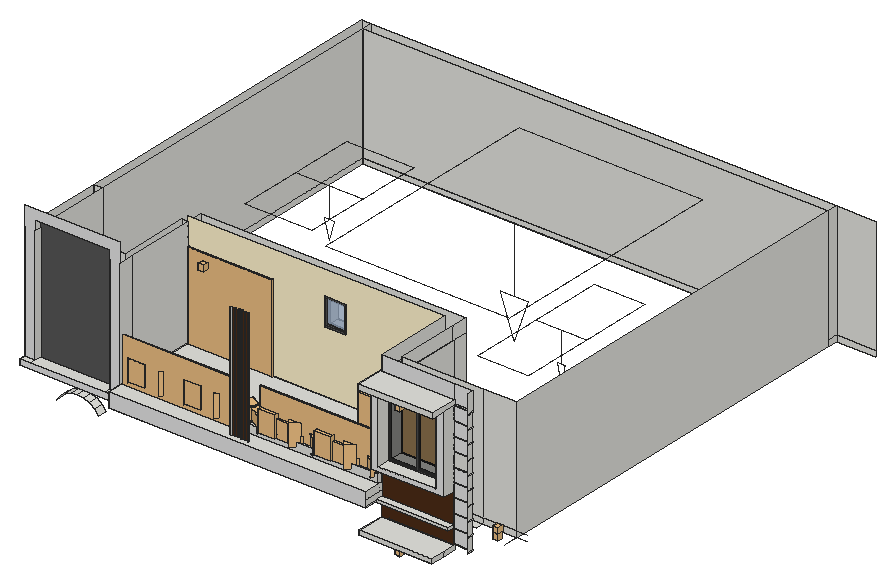
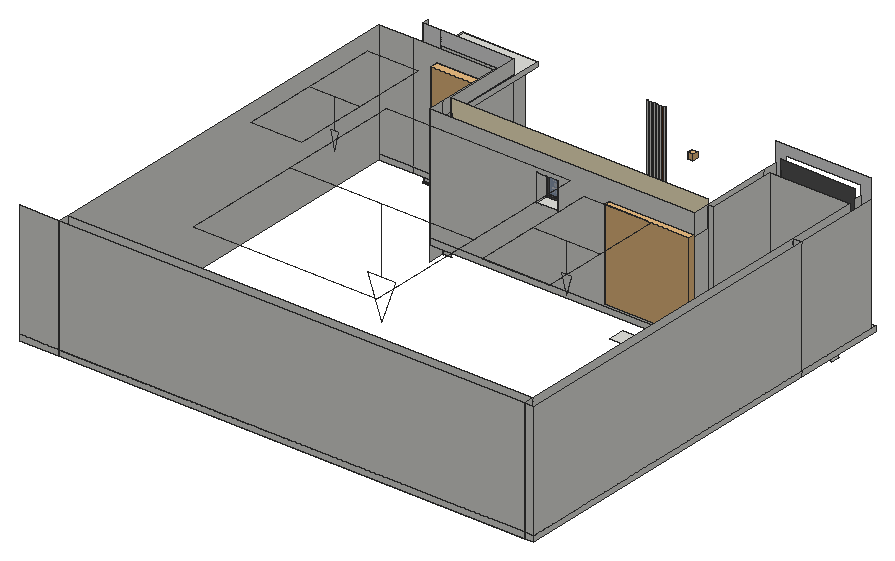
# SketchUp Ruby script. Lengths in inches.
U = 1.inch
M = Sketchup.active_model
def pt(a) = Geom::Point3d.new(a.map { |v| v * U })
def face(e, loops, mat)
  f = e.add_face(loops[0].map { |a| pt(a) })
  loops[1..].each { |l| e.add_face(l.map { |a| pt(a) }).erase! }
  f.material = f.back_material = mat if mat
  f
end
# faces: each face lists its corners as indices into pts; further lists are holes
def faces(e, pts, list, mat = nil) = list.each { |f| face(e, (f[0].is_a?(Array) ? f : [f]).map { |l| l.map { |i| pts[i] } }, mat) }
# xy, xz, yz: faces in a plane at the given z, y or x. An outline is a flat list of corners, or four numbers for a rectangle; further outlines are holes
def ring(l) = l.size == 4 ? [[l[0], l[1]], [l[2], l[1]], [l[2], l[3]], [l[0], l[3]]] : l.each_slice(2).to_a
def flat(e, list, mat, &to3) = list.each { |f| face(e, (f[0].is_a?(Array) ? f : [f]).map { |l| ring(l).map { |u, v| to3.(u, v) } }, mat) }
def xy(e, z, list, mat = nil) = flat(e, list, mat) { |x, y| [x, y, z] }
def xz(e, y, list, mat = nil) = flat(e, list, mat) { |x, z| [x, y, z] }
def yz(e, x, list, mat = nil) = flat(e, list, mat) { |y, z| [x, y, z] }
def lines(e, pts, list) = list.each { |a, b| e.add_line(pt(pts[a]), pt(pts[b])) }
# prism: a flat outline (further loops are holes) pulled along v
def prism(e, loops, v, mat = nil)
  f = face(e, loops, mat); d = Geom::Vector3d.new(v.map { |x| x * U })
  f.pushpull(f.normal.samedirection?(d) ? d.length : -d.length)
end
def box(e, o, s, mat = nil) = prism(e, [[o, [o[0] + s[0], o[1], o[2]], [o[0] + s[0], o[1] + s[1], o[2]], [o[0], o[1] + s[1], o[2]]]], [0, 0, s[2]], mat)
def at(x, y, z, deg = 0) = Geom::Transformation.translation(pt([x, y, z])) * Geom::Transformation.rotation(ORIGIN, Z_AXIS, deg.degrees)
def axes(o, x, y, z) = Geom::Transformation.new([*x, 0, *y, 0, *z, 0, *pt(o).to_a, 1])
def part(name) = M.definitions.add(name)
# library, detail: a bought-in or finely detailed component or shape, given as its bounding box
def library(name, o, s) = part(name).tap { |d| box(d.entities, o, s) }
def detail(e, o, s) = box(e.add_group.entities, o, s)
def put(e, d, t, mat = nil) = e.add_instance(d, t).tap { |i| i.material = mat if mat }
def group(e, t, mat = nil) = e.add_group.tap { |g| g.transformation = t; g.material = mat if mat }.entities
root = M.entities
M.materials.add("Glass_Tinted_Gray").color = [0, 0, 0]
M.materials["Glass_Tinted_Gray"].alpha = 0.125
M.materials.add("Material__1").color = [95, 70, 46]
M.materials.add("[0135_DarkGray]").color = [81, 81, 81]
M.materials.add("[Color D01]").color = [255, 242, 204]
M.materials.add("[Color M01]").color = [226, 226, 226]
M.materials.add("[Color M06]").color = [86, 86, 86]
M.materials.add("[Color_006]").color = [86, 86, 86]
M.materials.add("[Mirror 02]").color = [229, 229, 229]
M.materials.add("[Terrazzo Light Blue]").color = [196, 214, 227]
M.materials.add("[Translucent_Glass_Gray]1").color = [167, 187, 214]
M.materials["[Translucent_Glass_Gray]1"].alpha = 0.8
M.materials.add("[Wood Veneer 01]").color = [76, 44, 23]
c1 = library("SPOT",[0,0,1.68],[5.4375,5.4375,6.28])
c2 = library("Sliding Door",[0,0,0],[94.49,5.83,91.73])
c3 = library("Curtains",[0,0,0],[121.73,8.19,117.22])
c4 = part("glass-railing")
detail(c4.entities,[0,0,0],[1.26,75.59,33.1875])
c5 = library("Areca palm plant",[0,0,0],[49.1,36.6,54.46])
c6 = library("Group20\#1",[-20.81,-17.08,3.79],[39.86,39.43,37.51])
c7 = library("Group\#74",[-84.69,-90.07,-0.36],[176.51,175.13,171.4])
c8 = library("Group\#130",[-7.34,-1.2,0],[38.67,35.81,49.04])
c9 = library("Group38\#2",[14.01,28.44,-23.43],[18.58,18.32,38.89])
c10 = part("Group\#11")
put(c10.entities,c5,axes([-6.2,56.6,6.08],[0.45017,-0.56191,0],[0.66137,0.52986,0],[0,0,0.72]))
put(c10.entities,c5,axes([-6.2,158.41,6.08],[0.45017,-0.56191,0],[0.66137,0.52986,0],[0,0,0.72]))
put(c10.entities,c6,axes([18.97,181.79,4.77],[0,0.85,0],[-0.85,0,0],[0,0,0.85]))
put(c10.entities,c7,axes([14.93,71.3,6.05],[-0.04961,-0.08593,0],[0.08593,-0.04961,0],[0,0,0.10522]))
put(c10.entities,c7,axes([14.93,91.37,6.05],[-0.04961,-0.08593,0],[0.08593,-0.04961,0],[0,0,0.10522]))
put(c10.entities,c6,axes([18.97,79.98,4.77],[0,0.85,0],[-0.85,0,0],[0,0,0.85]))
put(c10.entities,c8,axes([24.9375,191.72,8],[0,0.79,0],[-0.79,0,0],[0,0,0.79]))
put(c10.entities,c7,axes([17.19,223.04,6.07],[-0.08133,-0.14087,0],[0.14087,-0.08133,0],[0,0,0.1725]))
put(c10.entities,c8,axes([24.9375,89.91,8],[0,0.79,0],[-0.79,0,0],[0,0,0.79]))
put(c10.entities,c7,axes([14.93,44.05,6.05],[-0.04961,-0.08593,0],[0.08593,-0.04961,0],[0,0,0.10522]))
put(c10.entities,c7,axes([14.93,145.87,6.05],[-0.04961,-0.08593,0],[0.08593,-0.04961,0],[0,0,0.10522]))
put(c10.entities,c9,axes([-4.1,100.66,28.17],[0.8848,0,0],[0,0.94674,0],[0,0,0.85826]))
put(c10.entities,c7,axes([14.93,173.12,6.05],[-0.04961,-0.08593,0],[0.08593,-0.04961,0],[0,0,0.10522]))
put(c10.entities,c9,axes([-4.1,-1.15,28.17],[0.8848,0,0],[0,0.94674,0],[0,0,0.85826]))
put(c10.entities,c7,axes([17.19,121.23,6.07],[-0.08133,-0.14087,0],[0.14087,-0.08133,0],[0,0,0.1725]))
put(c10.entities,c7,axes([14.93,193.18,6.05],[-0.04961,-0.08593,0],[0.08593,-0.04961,0],[0,0,0.10522]))
put(c10.entities,c7,axes([17.19,15.79,6.07],[-0.08133,-0.14087,0],[0.14087,-0.08133,0],[0,0,0.1725]))
g1 = group(c10.entities,at(0,0,0))
xy(g1,0,[[0,0,6,234.8],[30,0,36,234.8]])
xy(g1,3,[[6,0,30,234.8]])
xy(g1,7,[[6,5,30,229.8]],"Material__1")
xy(g1,15,[[[0,0,36,234.8],[6,5,30,229.8]]])
xz(g1,0,[[0,0,6,0,6,3,30,3,30,0,36,0,36,15,0,15]])
xz(g1,5,[[6,7,30,15]])
xz(g1,229.8,[[6,7,30,15]])
xz(g1,234.8,[[0,0,0,15,36,15,36,0,30,0,30,3,6,3,6,0]])
yz(g1,0,[[0,0,234.8,15]])
yz(g1,6,[[0,0,234.8,3],[5,7,229.8,15]])
yz(g1,30,[[0,0,234.8,3],[5,7,229.8,15]])
yz(g1,36,[[0,0,234.8,15]])
c11 = library("Flora+17",[-57.52,158.6,-38.64],[66.99,62.88,77.28])
c12 = part("Group211\#1")
p = [[0,0,0],[0,0,-68.24],[-14.65,0,-68.24],[95.41,-125.51,0],[-95.41,-125.51,0],[95.41,125.51,0],
  [95.41,0,0],[-95.41,125.51,0],[14.65,0,-68.24],[-95.41,0,0],[0,0,-110.46]]
lines(c12.entities,p,[[0,1],[1,2],[3,4],[5,6],[7,5],[1,8],[9,0],[0,6],[8,10],[4,9],[6,3],[2,10],
  [9,7]])
c13 = part("Rectangle Light")
put(c13.entities,c12,at(0,0,0))
c14 = part("PENTEK_RP Fineline 50S_Sliding_DoorCase_E1")
box(c14.entities,[0,0,0],[1.51,3.66,99.27],"[0135_DarkGray]")
c15 = part("PENTEK_RP Fineline 50S_SlidingDooe_Case_E2")
box(c15.entities,[0,0,0],[96.25,3.66,1.51],"[0135_DarkGray]")
c16 = part("pentek_RP Fineline 50S_SlidingDoor_Case")
put(c16.entities,c14,at(97.76,0,0))
put(c16.entities,c15,at(1.51,0,0))
put(c16.entities,c14,at(0,0,0))
put(c16.entities,c15,at(1.51,0,97.76))
c17 = part("PENTEK_RP Fineline 50S_SlidingDoor_GlazingBead_2")
box(c17.entities,[0,0,0],[0.56,0.59,94.39],"[0135_DarkGray]")
c18 = part("PENTEK_RP Fineline 50S_SlidingDoor_Glass")
box(c18.entities,[0,0,0],[46.58,0.16,94.39],"Glass_Tinted_Gray")
c19 = part("PENTEK_RP Fineline 50S_SlidingDoor_GlazingBead")
box(c19.entities,[0,0,0],[45.47,0.59,0.56],"[0135_DarkGray]")
c20 = part("PENTEK_RP Fineline 50S_SlidingDoor_Leaf_E1")
xy(c20.entities,0,[[0,0,0.93,1.97],[0.93,1.57,1.49,1.97]],"[0135_DarkGray]")
xy(c20.entities,96.25,[[0,0,0.93,0,0.93,1.57,1.49,1.57,1.49,1.97,0,1.97]],"[0135_DarkGray]")
xz(c20.entities,0,[[0,0,0.93,96.25]],"[0135_DarkGray]")
xz(c20.entities,1.57,[[0.93,0,1.49,95.32],[0.93,95.32,1.49,96.25]],"[0135_DarkGray]")
xz(c20.entities,1.97,[[0,0,1.49,96.25]],"[0135_DarkGray]")
yz(c20.entities,0,[[0,0,1.97,96.25]],"[0135_DarkGray]")
yz(c20.entities,0.93,[[0,0,1.57,0.93],[0,0.93,1.57,95.32],[0,95.32,1.57,96.25]],"[0135_DarkGray]")
yz(c20.entities,1.49,[[1.57,0,1.97,95.32],[1.57,95.32,1.97,96.25]],"[0135_DarkGray]")
c21 = part("PENTEK_RP Fineline 50S_SlidingDoor_Leaf_E2")
xy(c21.entities,0,[[0,0,0,1.57,0.56,1.57,0.56,1.97,46.02,1.97,46.02,1.57,46.58,1.57,46.58,0]],"[0135_DarkGray]")
xy(c21.entities,0.93,[[0,0,46.58,1.57]],"[0135_DarkGray]")
xy(c21.entities,1.49,[[0.56,1.57,46.02,1.97]],"[0135_DarkGray]")
xz(c21.entities,0,[[0,0,46.58,0.93]],"[0135_DarkGray]")
xz(c21.entities,1.57,[[0,0,0.56,0.93],[46.02,0,46.58,0.93],[0.56,0.93,46.02,1.49]],"[0135_DarkGray]")
xz(c21.entities,1.97,[[0.56,0,46.02,1.49]],"[0135_DarkGray]")
yz(c21.entities,0,[[0,0,1.57,0.93]],"[0135_DarkGray]")
yz(c21.entities,0.56,[[1.57,0,1.97,0.93],[1.57,0.93,1.97,1.49]],"[0135_DarkGray]")
yz(c21.entities,46.02,[[1.57,0,1.97,0.93],[1.57,0.93,1.97,1.49]],"[0135_DarkGray]")
yz(c21.entities,46.58,[[0,0,1.57,0.93]],"[0135_DarkGray]")
c22 = part("PENTEK_RP Fineline S_SlidingDoor_Leaf1")
put(c22.entities,c17,at(0.93,0,0.93))
put(c22.entities,c17,at(46.96,0,0.93))
put(c22.entities,c18,at(1.49,1.42,0.93))
put(c22.entities,c19,at(1.49,0,0.93))
put(c22.entities,c18,at(1.49,0.59,0.93),"[Terrazzo Light Blue]")
put(c22.entities,c20,at(0,0,0))
put(c22.entities,c20,axes([48.44,0,0],[-1,0,0],[0,1,0],[0,0,1]))
put(c22.entities,c21,axes([0.93,0,96.25],[1,0,0],[0,1,0],[0,0,-1]))
put(c22.entities,c21,at(0.93,0,0))
put(c22.entities,c19,at(1.49,0,94.77))
c23 = part("PENTEK_RP Fineline 50S_SlidingDoor_Leaf2")
put(c23.entities,c18,at(1.49,1.42,0.93))
put(c23.entities,c19,at(1.49,0,94.77))
put(c23.entities,c17,at(46.96,0,0.93))
put(c23.entities,c18,at(1.49,0.59,0.93),"[Mirror 02]")
put(c23.entities,c17,at(0.93,0,0.93))
put(c23.entities,c20,at(0,0,0))
put(c23.entities,c20,axes([48.44,0,0],[-1,0,0],[0,1,0],[0,0,1]))
put(c23.entities,c19,at(1.49,0,0.93))
put(c23.entities,c21,axes([0.93,0,96.25],[1,0,0],[0,1,0],[0,0,-1]))
put(c23.entities,c21,at(0.93,0,0))
c24 = part("PENTEK - Slimmest Steel Sliding Door / Window\#1")
put(c24.entities,c16,at(0,-1.88,-0.09))
put(c24.entities,c22,at(1.51,-2.27,1.42))
put(c24.entities,c23,at(49.32,-0.3,1.42))
c25 = part("Group215\#1")
p = [[0,0,0],[0,0,-31.53],[-4.05,0,-31.53],[26.38,-75.71,0],[-26.38,-75.71,0],[26.38,75.71,0],
  [26.38,0,0],[-26.38,75.71,0],[4.05,0,-31.53],[-26.38,0,0],[0,0,-51.04]]
lines(c25.entities,p,[[0,1],[1,2],[3,4],[5,6],[7,5],[1,8],[9,0],[0,6],[8,10],[4,9],[6,3],[2,10],
  [9,7]])
c26 = part("Rectangle Light\#2")
put(c26.entities,c25,at(0,0,0))
c27 = part("Group213\#1")
p = [[0,0,0],[0,0,-31.25],[-5.375,0,-31.25],[34.99,-66.18,0],[-34.99,-66.18,0],[34.99,66.18,0],
  [34.99,0,0],[-34.99,66.18,0],[5.375,0,-31.25],[-34.99,0,0],[0,0,-50.59]]
lines(c27.entities,p,[[0,1],[1,2],[3,4],[5,6],[7,5],[1,8],[9,0],[0,6],[8,10],[4,9],[6,3],[2,10],
  [9,7]])
c28 = part("Rectangle Light\#1")
put(c28.entities,c27,at(0,0,0))
c29 = part("BIC_Bike Shop - Window - Small")
xy(c29.entities,-8,[[[0,0,36,36],[2,2,34,34]]],"[Color_006]")
xy(c29.entities,-4,[[2,2,34,34]],"[Translucent_Glass_Gray]1")
xy(c29.entities,0,[[[0,0,36,36],[2,2,34,34]]],"[Color_006]")
xz(c29.entities,0,[[0,-8,36,0]],"[Color_006]")
xz(c29.entities,2,[[2,-8,34,-4],[2,-4,34,0]],"[Color_006]")
xz(c29.entities,34,[[2,-8,34,-4],[2,-4,34,0]],"[Color_006]")
xz(c29.entities,36,[[0,-8,36,0]],"[Color_006]")
yz(c29.entities,0,[[0,-8,36,0]],"[Color_006]")
yz(c29.entities,2,[[2,-8,34,-4],[2,-4,34,0]],"[Color_006]")
yz(c29.entities,34,[[2,-8,34,-4],[2,-4,34,0]],"[Color_006]")
yz(c29.entities,36,[[0,-8,36,0]],"[Color_006]")
prism(root,[[[693.82,242.98,360.97],[694.53,243.27,360.97],[695.29,243.375,360.97],[696.05,243.27,360.97],[696.76,242.98,360.97],[697.37,242.51,360.97],[697.84,241.91,360.97],[698.13,241.2,360.97],[698.23,240.4375,360.97],[698.13,239.68,360.97],[697.84,238.97,360.97],[697.37,238.36,360.97],[696.76,237.89,360.97],[696.05,237.6,360.97],[695.29,237.5,360.97],[694.53,237.6,360.97],[693.82,237.89,360.97],[693.22,238.36,360.97],[692.75,238.97,360.97],[692.45,239.68,360.97],[692.35,240.4375,360.97],[692.45,241.2,360.97],[692.75,241.91,360.97],[693.22,242.51,360.97]]],[0,0,0.6875])
xy(root,358.37,[[664.71,249.36,724.59,263.24]])
xy(root,361.12,[[657.09,234.3,732.9,249.36],[657.09,249.36,732.9,263.24]])
xy(root,361.75,[[390.34,345.71,390.9,362.65],[390.9,345.71,478.4,362.65]])
xy(root,365.68,[[657.09,234.3,732.9,263.24]])
xy(root,367.16,[[733.09,261.68,751.93,263.24]])
xy(root,367.49,[[665.11,271.58,724.59,279.2],[664.05,279.2,665.11,345.71]])
xy(root,368.1,[[733.09,261.68,751.93,263.24]])
xy(root,381.46,[[733.09,261.68,751.93,263.24]])
xy(root,382.4,[[733.09,261.68,751.93,263.24]])
xy(root,382.6875,[[732.93,254.0625,657.09,255.62,657.09,263.24,733.09,261.68],[657.09,255.62,656.93,255.625,657.09,263.24]])
xy(root,382.6875,[[[390.34,242.18,390.34,345.71,657.09,345.71,657.09,263.24,656.93,255.625,657.09,255.62,657.09,242.18],[447.91,289.875,449.21,289.96,450.45,290.37,451.53,291.09,452.4,292.07,452.98,293.24,453.24,294.52,453.16,295.82,452.75,297.06,452.03,298.14,451.05,299.01,449.88,299.59,448.6,299.85,447.3,299.77,446.0625,299.36,444.97,298.64,444.11,297.66,443.53,296.49,443.27,295.21,443.35,293.91,443.76,292.67,444.48,291.58,445.46,290.72,446.625,290.14],[595.53,289.875,596.83,289.96,598.07,290.37,599.16,291.09,600.02,292.07,600.61,293.24,600.87,294.52,600.79,295.82,600.37,297.06,599.65,298.14,598.67,299.01,597.51,299.59,596.23,299.85,594.92,299.77,593.6875,299.36,592.6,298.64,591.73,297.66,591.15,296.49,590.89,295.21,590.97,293.91,591.39,292.67,592.11,291.58,593.08,290.72,594.25,290.14]]],"[Wood Veneer 01]")
xy(root,383.75,[[447.91,289.875,446.625,290.14,445.46,290.72,444.48,291.58,443.76,292.67,443.35,293.91,443.27,295.21,443.53,296.49,444.11,297.66,444.97,298.64,446.0625,299.36,447.3,299.77,448.6,299.85,449.88,299.59,451.05,299.01,452.03,298.14,452.75,297.06,453.16,295.82,453.24,294.52,452.98,293.24,452.4,292.07,451.53,291.09,450.45,290.37,449.21,289.96],[595.53,289.875,594.25,290.14,593.08,290.72,592.11,291.58,591.39,292.67,590.97,293.91,590.89,295.21,591.15,296.49,591.73,297.66,592.6,298.64,593.6875,299.36,594.92,299.77,596.23,299.85,597.51,299.59,598.67,299.01,599.65,298.14,600.37,297.06,600.79,295.82,600.87,294.52,600.61,293.24,600.02,292.07,599.16,291.09,598.07,290.37,596.83,289.96]])
xy(root,384,[[292.06,249.93,302.78,256.61],[302.78,249.93,380.53,263.24],[380.53,249.93,390.34,256.61],[292.06,256.61,292.06,345.71,301.28,345.71,301.28,272.46,383.72,272.46,383.72,345.71,390.34,345.71,390.34,256.61,380.53,256.61,380.53,263.24,302.78,263.24,302.78,256.61],[665.11,271.58,749.59,279.2],
  [292.06,345.71,301.28,694.43],[301.28,683.75,784.56,694.43]])
xy(root,385.39,[[732.93,254.0625,733.09,261.68,657.09,263.24,656.93,255.625]])
xy(root,389.875,[[511.65,248.63,512.53,250.63],[529.78,248.63,530.65,250.63],[512.53,249.32,515.36,250.63],[516,249.32,518.83,250.63],[519.47,249.32,522.3,250.63],
  [522.9375,249.32,525.77,250.63],[526.41,249.32,529.24,250.63]])
xy(root,390,[[292.06,249.93,302.78,256.61],[302.78,249.93,380.53,263.24],[380.53,249.93,390.34,256.61],[292.06,256.61,292.06,345.71,301.28,345.71,301.28,272.46,383.72,272.46,383.72,345.71,390.34,345.71,390.34,256.61,380.53,256.61,380.53,263.24,302.78,263.24,302.78,256.61],[292.06,345.71,301.28,694.43],
  [301.28,683.75,784.56,694.43]])
xy(root,394.625,[[511.65,248.63,512.53,250.63],[529.78,248.63,530.65,250.63],[512.53,249.32,515.36,250.63],[516,249.32,518.83,250.63],[519.47,249.32,522.3,250.63],
  [522.9375,249.32,525.77,250.63],[526.41,249.32,529.24,250.63],[390.34,345.71,390.9,362.65],[390.9,345.71,478.4,362.65]])
xy(root,395.76,[[733.09,261.68,751.93,263.24]])
xy(root,396.7,[[733.09,261.68,751.93,263.24]])
xy(root,397.4375,[[390.34,242.18,657.09,345.71]])
xy(root,410.06,[[733.09,261.68,751.93,263.24]])
xy(root,411,[[733.09,261.68,751.93,263.24]])
xy(root,416.38,[[657.09,249.36,733.09,263.24]])
xy(root,420.98,[[664.71,249.36,724.59,263.24],[664.71,263.24,724.59,279.2],[665.11,279.2,665.73,345.71]])
xy(root,424.36,[[733.09,261.68,751.93,263.24]])
xy(root,425.3,[[733.09,261.68,751.93,263.24]])
xy(root,438.66,[[733.09,261.68,751.93,263.24]])
xy(root,439.59,[[733.09,261.68,751.93,263.24]])
xy(root,452.96,[[733.09,261.68,751.93,263.24]])
xy(root,453.89,[[733.09,261.68,751.93,263.24]])
xy(root,462.0625,[[531.79,345.71,553.72,362.65]])
xy(root,467.25,[[733.09,261.68,751.93,263.24]])
xy(root,468.19,[[733.09,261.68,751.93,263.24]])
xy(root,481.55,[[733.09,261.68,751.93,263.24]])
xy(root,482.49,[[733.09,261.68,751.93,263.24]])
xy(root,487.75,[[390.34,345.71,390.9,362.65],[390.9,345.71,478.4,362.65]])
xy(root,490.4375,[[531.79,345.71,553.72,362.65]])
xy(root,495.67,[[664.71,263.24,724.59,279.2],[665.11,279.2,665.73,345.71]])
xy(root,495.67,[[664.71,249.36,724.59,263.24]],"[Color M01]")
xy(root,495.85,[[655.65,249.36,657.09,345.71],[657.09,249.36,733.09,263.24],[733.09,261.68,751.93,263.24]])
xy(root,495.85,[[[655.65,234.3,733.09,249.36],[695.29,237.6875,696,237.78,696.67,238.06,697.24,238.49,697.67,239.0625,697.95,239.73,698.04,240.4375,697.95,241.15,697.67,241.8125,697.24,242.38,696.67,242.82,696,243.09,695.29,243.1875,694.58,243.09,693.92,242.82,693.35,242.38,692.91,241.8125,692.64,241.15,692.54,240.4375,692.64,239.73,692.91,239.0625,693.35,238.49,693.92,238.06,694.58,237.78]]],"[Color M01]")
xy(root,496.41,[[695.29,237.6875,694.58,237.78,693.92,238.06,693.35,238.49,692.91,239.0625,692.64,239.73,692.54,240.4375,692.64,241.15,692.91,241.8125,693.35,242.38,693.92,242.82,694.58,243.09,695.29,243.1875,696,243.09,696.67,242.82,697.24,242.38,697.67,241.8125,697.95,241.15,698.04,240.4375,697.95,239.73,697.67,239.0625,697.24,238.49,696.67,238.06,696,237.78]])
xy(root,501.16,[[655.65,234.3,733.09,234.3,733.09,263.24,657.09,263.24,657.09,345.71,655.65,345.71]])
xz(root,234.3,[[657.09,361.12,732.9,365.68],[655.65,495.85,733.09,501.16]])
xz(root,242.18,[[390.34,382.6875,657.09,397.4375]],"[Color M01]")
xz(root,248.63,[[511.65,394.625,512.53,515.875],[529.78,394.625,530.65,515.875]])
xz(root,249.32,[[512.53,394.625,515.36,515.875],[516,394.625,518.83,515.875],[519.47,394.625,522.3,515.875],[522.9375,394.625,525.77,515.875],[526.41,394.625,529.24,515.875]],"[Wood Veneer 01]")
xz(root,249.36,[[[657.09,416.38,733.09,495.85],[664.71,420.98,724.59,495.67]]],"[Color M01]")
xz(root,249.93,[[292.06,384,390.34,390]],"[Color M01]")
xz(root,256.61,[[292.06,390,302.78,390,302.78,519.6875,380.53,519.6875,380.53,390,390.34,390,390.34,530.25,292.06,530.25]],"[Color M01]")
xz(root,261.68,[[733.09,439.59,751.93,452.96]])
xz(root,261.68,[[733.09,368.1,751.93,381.46],[733.09,382.4,751.93,395.76],[733.09,396.7,751.93,410.06],[733.09,411,751.93,424.36],[733.09,425.3,751.93,438.66],
  [733.09,453.89,751.93,467.25],[733.09,468.19,751.93,481.55],[733.09,482.49,751.93,495.85]],"[Color M01]")
xz(root,263.24,[[664.71,358.37,724.59,361.12],[657.09,361.12,664.71,365.68],[664.71,361.12,724.59,365.68],[724.59,361.12,732.9,365.68],[733.09,367.16,751.93,368.1],
  [733.09,381.46,751.93,382.4],[733.09,395.76,751.93,396.7],[733.09,410.06,751.93,411],[[657.09,416.38,733.09,495.85],[664.71,420.98,724.59,495.67]],[733.09,424.36,751.93,425.3],
  [733.09,438.66,751.93,439.59],[733.09,452.96,751.93,453.89],[733.09,467.25,751.93,468.19],[733.09,481.55,751.93,482.49],[657.09,495.85,733.09,501.16],
  [733.09,495.85,751.93,496.79]])
xz(root,263.24,[[733.09,496.79,751.93,515.875],[657.09,501.16,733.09,515.875]],"[Color M01]")
xz(root,263.24,[[302.78,390,380.53,519.6875]],"[Color M06]")
xz(root,263.24,[[657.09,365.68,732.9,365.68,732.9,367.82,733.09,367.82,733.09,416.38,657.09,416.38]],"[Wood Veneer 01]")
xz(root,272.46,[[301.28,384,383.72,390],[301.28,390,383.72,510]])
xz(root,279.2,[[665.11,384,749.59,390],[749.59,384,784.56,390],[665.11,390,665.11,420.98,724.59,420.98,724.59,495.67,665.11,495.67,665.11,510,749.59,510,749.59,390],[749.59,390,784.56,510],[664.71,420.98,665.11,495.67],
  [665.11,420.98,665.73,495.67]])
xz(root,345.71,[[657.09,367.82,664.71,377.4375],[390.34,382.6875,657.09,384],[292.06,384,301.28,390],[383.72,384,390.34,390],[292.06,390,301.28,510],
  [383.72,390,390.34,510],[390.34,390,657.09,390,657.09,397.4375,478.4,397.4375,478.4,394.625,390.34,394.625],[390.34,394.625,390.9,397.4375],[390.9,394.625,478.4,397.4375],[390.34,397.4375,390.9,487.75],
  [665.11,420.98,665.73,495.67]])
xz(root,345.71,[[[478.4,397.4375,657.09,397.4375,657.09,495.85,655.65,495.85,655.65,501.16,657.09,501.16,657.09,515.875,390.34,515.875,390.34,487.75,478.4,487.75],[531.79,462.0625,553.72,490.4375]]],"[Color D01]")
xz(root,362.65,[[390.34,384,665.11,390],[[390.34,390,390.34,394.625,478.4,394.625,478.4,487.75,390.34,487.75,390.34,510,665.11,510,665.11,390],[531.79,462.0625,553.72,490.4375]],[390.34,394.625,390.9,487.75]])
xz(root,683.75,[[301.28,384,784.56,390],[301.28,390,784.56,510]])
xz(root,694.43,[[292.06,384,301.28,390],[301.28,384,784.56,390],[784.56,384,825.43,390],[292.06,390,301.28,510],[301.28,390,784.56,510],
  [784.56,390,825.43,510]])
yz(root,292.06,[[249.93,384,345.71,390],[345.71,384,694.43,390],[256.61,390,345.71,510],[345.71,390,694.43,510]])
yz(root,301.28,[[272.46,384,345.71,390],[345.71,384,683.75,390],[683.75,384,694.43,390],[272.46,390,345.71,510],[345.71,390,683.75,510],
  [683.75,390,694.43,510]])
yz(root,302.78,[[256.61,390,263.24,510]])
yz(root,380.53,[[256.61,390,263.24,510]])
yz(root,383.72,[[272.46,384,345.71,390],[272.46,390,345.71,510]])
yz(root,390.34,[[345.71,361.75,362.65,384],[242.18,382.6875,256.61,384],[256.61,382.6875,272.46,384],[272.46,382.6875,345.71,384],[242.18,384,249.93,390],
  [249.93,384,272.46,390],[272.46,384,345.71,390],[345.71,384,362.65,390],[242.18,390,256.61,397.4375],[256.61,390,272.46,397.4375],
  [272.46,390,345.71,397.4375],[345.71,390,362.65,394.625],[345.71,394.625,362.65,487.75],[256.61,397.4375,272.46,510],[272.46,397.4375,345.71,510],
  [345.71,487.75,362.65,510]])
yz(root,390.9,[[345.71,394.625,362.65,487.75]])
yz(root,478.4,[[345.71,394.625,362.65,487.75]])
yz(root,512.53,[[248.63,394.625,249.32,515.875]])
yz(root,515.36,[[249.32,394.625,250.63,515.875]])
yz(root,516,[[249.32,394.625,250.63,515.875]])
yz(root,518.83,[[249.32,394.625,250.63,515.875]])
yz(root,519.47,[[249.32,394.625,250.63,515.875]])
yz(root,522.3,[[249.32,394.625,250.63,515.875]])
yz(root,522.9375,[[249.32,394.625,250.63,515.875]])
yz(root,525.77,[[249.32,394.625,250.63,515.875]])
yz(root,526.41,[[249.32,394.625,250.63,515.875]])
yz(root,529.24,[[249.32,394.625,250.63,515.875]])
yz(root,529.78,[[248.63,394.625,250.63,515.875]])
yz(root,531.79,[[345.71,462.0625,362.65,490.4375]])
yz(root,553.72,[[345.71,462.0625,362.65,490.4375]])
yz(root,655.65,[[234.3,495.85,345.71,501.16]])
yz(root,657.09,[[234.3,361.12,263.24,365.68],[242.18,382.6875,263.24,384],[263.24,382.6875,345.71,384],[242.18,384,263.24,390],[242.18,390,263.24,397.4375],
  [263.24,390,345.71,397.4375],[263.24,397.4375,345.71,495.85],[249.36,416.38,263.24,495.85],[263.24,495.85,345.71,501.16],[263.24,501.16,345.71,515.875]])
yz(root,664.71,[[249.36,420.98,263.24,495.67],[263.24,420.98,279.2,495.67]])
yz(root,665.11,[[271.58,367.49,279.2,384],[279.2,367.49,345.71,384],[345.71,367.49,362.65,384],[279.2,384,345.71,390],[345.71,384,362.65,390],
  [279.2,390,345.71,420.98],[345.71,390,362.65,420.98],[279.2,420.98,345.71,495.67],[345.71,420.98,362.65,495.67],[279.2,495.67,345.71,510],
  [345.71,495.67,362.65,510]])
yz(root,665.73,[[279.2,420.98,345.71,495.67]])
yz(root,724.59,[[249.36,420.98,263.24,495.67],[263.24,420.98,279.2,495.67]])
yz(root,732.9,[[234.3,361.12,249.36,365.68],[249.36,361.12,263.24,365.68]])
yz(root,733.09,[[261.68,367.82,263.24,368.1],[261.68,368.1,263.24,381.46],[261.68,382.4,263.24,395.76],[261.68,396.7,263.24,410.06],[261.68,411,263.24,416.38],
  [249.36,416.38,261.68,416.38,261.68,424.36,263.24,424.36,263.24,425.3,261.68,425.3,261.68,438.66,263.24,438.66,263.24,439.59,261.68,439.59,261.68,452.96,263.24,452.96,263.24,453.89,261.68,453.89,261.68,467.25,263.24,467.25,263.24,468.19,261.68,468.19,261.68,481.55,263.24,481.55,263.24,482.49,261.68,482.49,261.68,495.85,249.36,495.85],[261.68,416.38,263.24,424.36],[261.68,425.3,263.24,438.66],[261.68,439.59,263.24,452.96],[261.68,453.89,263.24,467.25],
  [261.68,468.19,263.24,481.55],[261.68,482.49,263.24,495.85],[234.3,495.85,263.24,501.16]])
yz(root,751.93,[[256.61,367.16,263.24,368.1],[256.61,368.1,261.68,381.46],[256.61,381.46,263.24,382.4],[256.61,382.4,261.68,395.76],[256.61,395.76,263.24,396.7],
  [256.61,396.7,261.68,410.06],[256.61,410.06,263.24,411],[256.61,411,261.68,424.36],[256.61,424.36,263.24,425.3],[256.61,425.3,261.68,438.66],
  [256.61,438.66,263.24,439.59],[256.61,439.59,261.68,452.96],[256.61,452.96,263.24,453.89],[256.61,453.89,261.68,467.25],[256.61,467.25,263.24,468.19],
  [256.61,468.19,261.68,481.55],[256.61,481.55,263.24,482.49],[256.61,482.49,261.68,495.85],[256.61,495.85,263.24,496.79],[256.61,496.79,263.24,515.875]])
yz(root,784.56,[[279.2,384,683.75,510],[683.75,384,694.43,390],[683.75,390,694.43,510]])
p = [[324,263.24,361.09],[320.07,263.24,355.97],[320.07,272.46,355.97],[324,272.46,361.09],[362.9375,263.24,355.97],[359,263.24,361.09],
  [359,272.46,361.09],[362.9375,272.46,355.97],[329.125,263.24,365.03],[329.125,272.46,365.03],[353.875,263.24,365.03],[353.875,272.46,365.03],
  [335.1,263.24,367.5],[335.1,272.46,367.5],[347.91,263.24,367.5],[347.91,272.46,367.5],[341.5,263.24,368.34],[341.5,272.46,368.34],
  [656.93,255.625,384],[656.93,255.625,382.6875],[657.09,255.62,382.6875],[732.93,254.0625,382.6875],[732.93,254.0625,385.39],[656.93,255.625,385.39],
  [733.09,261.68,382.6875],[733.09,261.68,385.39],[657.09,263.24,384],[657.09,263.24,382.6875],[447.91,289.875,382.6875],[446.625,290.14,382.6875],
  [446.625,290.14,383.75],[447.91,289.875,383.75],[449.21,289.96,382.6875],[449.21,289.96,383.75],[595.53,289.875,382.6875],[594.25,290.14,382.6875],
  [594.25,290.14,383.75],[595.53,289.875,383.75],[596.83,289.96,382.6875],[596.83,289.96,383.75],[450.45,290.37,382.6875],[450.45,290.37,383.75],
  [598.07,290.37,382.6875],[598.07,290.37,383.75],[445.46,290.72,382.6875],[445.46,290.72,383.75],[593.08,290.72,382.6875],[593.08,290.72,383.75],
  [451.53,291.09,382.6875],[451.53,291.09,383.75],[599.16,291.09,382.6875],[599.16,291.09,383.75],[444.48,291.58,382.6875],[444.48,291.58,383.75],
  [592.11,291.58,382.6875],[592.11,291.58,383.75],[452.4,292.07,382.6875],[452.4,292.07,383.75],[600.02,292.07,382.6875],[600.02,292.07,383.75],
  [443.76,292.67,382.6875],[443.76,292.67,383.75],[591.39,292.67,382.6875],[591.39,292.67,383.75],[452.98,293.24,382.6875],[452.98,293.24,383.75],
  [600.61,293.24,382.6875],[600.61,293.24,383.75],[443.35,293.91,382.6875],[443.35,293.91,383.75],[590.97,293.91,382.6875],[590.97,293.91,383.75],
  [453.24,294.52,382.6875],[453.24,294.52,383.75],[600.87,294.52,382.6875],[600.87,294.52,383.75],[443.27,295.21,382.6875],[443.27,295.21,383.75],
  [590.89,295.21,382.6875],[590.89,295.21,383.75],[453.16,295.82,382.6875],[453.16,295.82,383.75],[600.79,295.82,382.6875],[600.79,295.82,383.75],
  [443.53,296.49,382.6875],[443.53,296.49,383.75],[591.15,296.49,382.6875],[591.15,296.49,383.75],[452.75,297.06,382.6875],[452.75,297.06,383.75],
  [600.37,297.06,382.6875],[600.37,297.06,383.75],[444.11,297.66,382.6875],[444.11,297.66,383.75],[591.73,297.66,382.6875],[591.73,297.66,383.75],
  [452.03,298.14,382.6875],[452.03,298.14,383.75],[599.65,298.14,382.6875],[599.65,298.14,383.75],[444.97,298.64,382.6875],[444.97,298.64,383.75],
  [592.6,298.64,382.6875],[592.6,298.64,383.75],[451.05,299.01,382.6875],[451.05,299.01,383.75],[598.67,299.01,382.6875],[598.67,299.01,383.75],
  [446.0625,299.36,382.6875],[446.0625,299.36,383.75],[593.6875,299.36,382.6875],[593.6875,299.36,383.75],[449.88,299.59,382.6875],[449.88,299.59,383.75],
  [597.51,299.59,382.6875],[597.51,299.59,383.75],[447.3,299.77,382.6875],[447.3,299.77,383.75],[594.92,299.77,382.6875],[594.92,299.77,383.75],
  [448.6,299.85,382.6875],[448.6,299.85,383.75],[596.23,299.85,382.6875],[596.23,299.85,383.75],[657.09,263.24,385.39],[695.29,237.6875,495.85],
  [694.58,237.78,495.85],[694.58,237.78,496.41],[695.29,237.6875,496.41],[696,237.78,495.85],[696,237.78,496.41],[693.92,238.06,495.85],
  [693.92,238.06,496.41],[696.67,238.06,495.85],[696.67,238.06,496.41],[693.35,238.49,495.85],[693.35,238.49,496.41],[697.24,238.49,495.85],
  [697.24,238.49,496.41],[692.91,239.0625,495.85],[692.91,239.0625,496.41],[697.67,239.0625,495.85],[697.67,239.0625,496.41],[692.64,239.73,495.85],
  [692.64,239.73,496.41],[697.95,239.73,495.85],[697.95,239.73,496.41],[692.54,240.4375,495.85],[692.54,240.4375,496.41],[698.04,240.4375,495.85],
  [698.04,240.4375,496.41],[692.64,241.15,495.85],[692.64,241.15,496.41],[697.95,241.15,495.85],[697.95,241.15,496.41],[692.91,241.8125,495.85],
  [692.91,241.8125,496.41],[697.67,241.8125,495.85],[697.67,241.8125,496.41],[693.35,242.38,495.85],[693.35,242.38,496.41],[697.24,242.38,495.85],
  [697.24,242.38,496.41],[693.92,242.82,495.85],[693.92,242.82,496.41],[696.67,242.82,495.85],[696.67,242.82,496.41],[694.58,243.09,495.85],
  [694.58,243.09,496.41],[696,243.09,495.85],[696,243.09,496.41],[695.29,243.1875,495.85],[695.29,243.1875,496.41],[784.56,279.2,384],
  [795.31,279.2,384],[784.56,263.24,384],[784.56,279.2,390],[795.31,279.2,390],[724.59,263.24,367.49],[724.59,271.58,367.49],
  [664.71,263.24,367.49],[664.71,279.2,367.49],[657.84,259.36,394.54],[657.84,259.36,394.38],[657.09,345.71,367.82],[655.46,345.71,367.82],
  [732.9,249.36,361.63],[733.09,249.36,361.63]]
faces(root,p,[[0,1,2,3],[4,5,6,7],[8,0,3,9],[5,10,11,6],[12,8,9,13],[10,14,15,11],[16,12,13,17],[14,16,17,15],
  [18,19,20,21,22,23],[24,25,22,21],[26,27,19,18],[28,29,30,31],[32,28,31,33],[34,35,36,37],[38,34,37,39],[40,32,33,41],
  [42,38,39,43],[29,44,45,30],[35,46,47,36],[48,40,41,49],[50,42,43,51],[44,52,53,45],[46,54,55,47],[56,48,49,57],
  [58,50,51,59],[52,60,61,53],[54,62,63,55],[64,56,57,65],[66,58,59,67],[60,68,69,61],[62,70,71,63],[72,64,65,73],
  [74,66,67,75],[68,76,77,69],[70,78,79,71],[80,72,73,81],[82,74,75,83],[76,84,85,77],[78,86,87,79],[88,80,81,89],
  [90,82,83,91],[84,92,93,85],[86,94,95,87],[96,88,89,97],[98,90,91,99],[92,100,101,93],[94,102,103,95],[104,96,97,105],
  [106,98,99,107],[100,108,109,101],[102,110,111,103],[112,104,105,113],[114,106,107,115],[108,116,117,109],[110,118,119,111],[120,112,113,121],
  [122,114,115,123],[116,120,121,117],[118,122,123,119],[124,26,18,23],[125,126,127,128],[129,125,128,130],[126,131,132,127],[133,129,130,134],
  [131,135,136,132],[137,133,134,138],[135,139,140,136],[141,137,138,142],[139,143,144,140],[145,141,142,146],[143,147,148,144],[149,145,146,150],
  [147,151,152,148],[153,149,150,154],[151,155,156,152],[157,153,154,158],[155,159,160,156],[161,157,158,162],[159,163,164,160],[165,161,162,166],
  [163,167,168,164],[169,165,166,170],[167,171,172,168],[171,169,170,172]])
lines(root,p,[[173,174],[175,173],[176,177],[178,179],[180,181],[182,183],[184,185],[186,187]])
put(root,c1,at(692.4,236.47,352.92))
put(root,c1,at(445.57,289.74,374.41))
put(root,c1,at(593.24,293.57,375.7))
put(root,c1,at(782.11,251.18,392.15))
put(root,c2,axes([390.9,344.49,394.625],[0.92604,0,0],[0,1,0],[0,0,1.01518]))
put(root,c3,axes([390.9,360.43,396.9],[0.71882,0,0],[0,1,0],[0,0,0.79]))
put(root,c4,axes([530.65,264.37,397.4375],[0,-1.29,0],[1.65356,0,0],[0,0,1.37437]))
put(root,c4,axes([390.34,260.57,397.4375],[0,-1.29,0],[1.60489,0,0],[0,0,1.38316]))
put(root,c10,axes([655.88,260.15,397.4375],[0,0.57,0],[-0.57,0,0],[0,0,0.57]))
put(root,c10,axes([520.94,260.15,397.4375],[0,0.57,0],[-0.57,0,0],[0,0,0.57]))
put(root,c11,axes([661.12,159.64,428],[0.78,0,0],[0,0.78,0],[0,0,0.78]))
put(root,c13,at(597.76,509.34,509.99,180))
put(root,c1,axes([787.47,251.75,407.94],[-1,0,0],[0,1,0],[0,0,-1]))
put(root,c24,axes([664.71,263.95,420.96],[0.6,0,0],[0,0.6,0],[0,0,0.75514]))
put(root,c3,axes([665.73,279.2,421.66],[0.4835,0,0],[0,1,0],[0,0,0.63137]))
put(root,c26,axes([738.38,394.79,509.99],[-1,0,0],[0,1,0],[0,0,1]))
put(root,c28,axes([442.42,463.63,509.99],[-1,0,0],[0,1,0],[0,0,1]))
put(root,c29,axes([531.76,345.71,462.0625],[0.61,0,0],[0,0,0.78819],[0,-0.61,0]))
put(root,c1,at(692.51,235.71,487.81))
put(root,c1,at(445.57,289.74,507.59))
